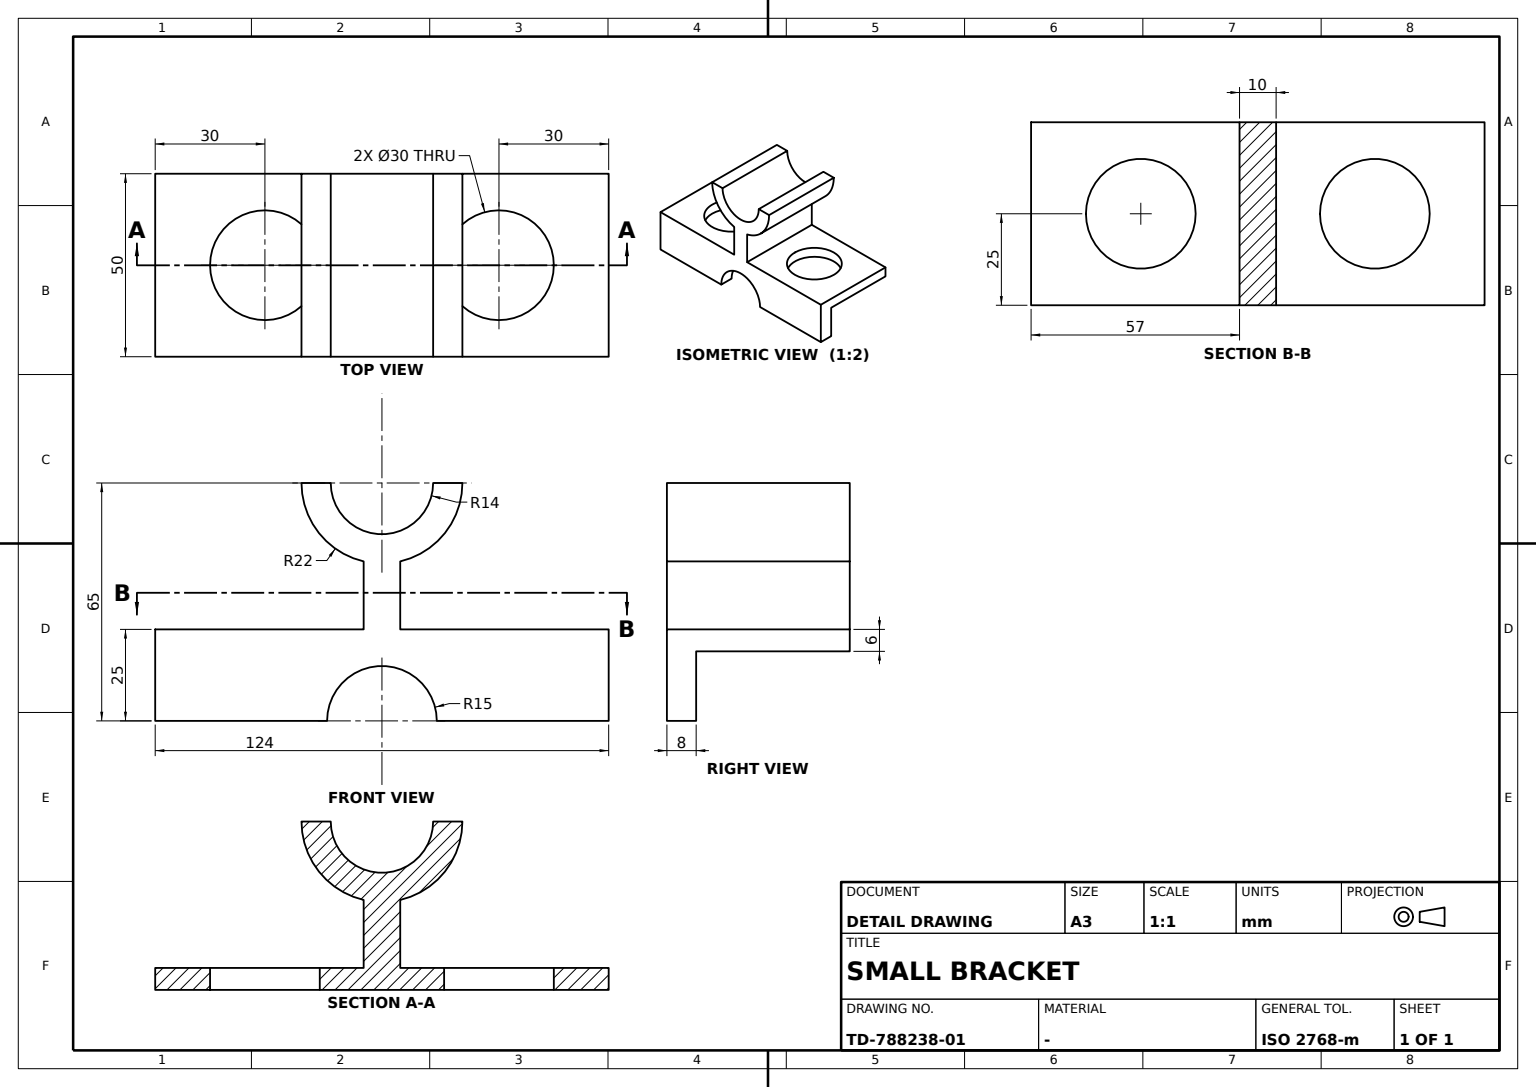
ISO-10303-21;
HEADER;
FILE_DESCRIPTION((''),'2;1');
FILE_NAME('','',(''),(''),'','','');
FILE_SCHEMA(('AUTOMOTIVE_DESIGN'));
ENDSEC;
DATA;
#1=APPLICATION_CONTEXT('');
#2=PRODUCT_CONTEXT('',#1,'mechanical');
#3=PRODUCT('','','',(#2));
#4=PRODUCT_DEFINITION_FORMATION('','',#3);
#5=PRODUCT_DEFINITION_CONTEXT('',#1,'design');
#6=PRODUCT_DEFINITION('','',#4,#5);
#7=PRODUCT_DEFINITION_SHAPE('','',#6);
#8=(LENGTH_UNIT()NAMED_UNIT(*)SI_UNIT(.MILLI.,.METRE.));
#9=(NAMED_UNIT(*)PLANE_ANGLE_UNIT()SI_UNIT($,.RADIAN.));
#10=(NAMED_UNIT(*)SI_UNIT($,.STERADIAN.)SOLID_ANGLE_UNIT());
#11=UNCERTAINTY_MEASURE_WITH_UNIT(LENGTH_MEASURE(0.005),#8,'distance_accuracy_value','');
#12=(GEOMETRIC_REPRESENTATION_CONTEXT(3)GLOBAL_UNCERTAINTY_ASSIGNED_CONTEXT((#11))GLOBAL_UNIT_ASSIGNED_CONTEXT((#8,#9,#10))REPRESENTATION_CONTEXT('',''));
#13=CARTESIAN_POINT('',(-62.,0.,25.));
#14=VERTEX_POINT('',#13);
#15=CARTESIAN_POINT('',(-5.,0.,25.));
#16=VERTEX_POINT('',#15);
#17=CARTESIAN_POINT('',(0.,0.,25.));
#18=DIRECTION('',(1.,0.,0.));
#19=VECTOR('',#18,1000.);
#20=LINE('',#17,#19);
#21=EDGE_CURVE('',#14,#16,#20,.T.);
#22=ORIENTED_EDGE('',*,*,#21,.T.);
#23=CARTESIAN_POINT('',(-5.,50.,25.));
#24=VERTEX_POINT('',#23);
#25=DIRECTION('',(0.,1.,0.));
#26=VECTOR('',#25,1000.);
#27=LINE('',#15,#26);
#28=EDGE_CURVE('',#16,#24,#27,.T.);
#29=ORIENTED_EDGE('',*,*,#28,.T.);
#30=CARTESIAN_POINT('',(-62.,50.,25.));
#31=VERTEX_POINT('',#30);
#32=CARTESIAN_POINT('',(0.,50.,25.));
#33=LINE('',#32,#19);
#34=EDGE_CURVE('',#31,#24,#33,.T.);
#35=ORIENTED_EDGE('',*,*,#34,.F.);
#36=LINE('',#13,#26);
#37=EDGE_CURVE('',#14,#31,#36,.T.);
#38=ORIENTED_EDGE('',*,*,#37,.F.);
#39=EDGE_LOOP('',(#22,#29,#35,#38));
#40=FACE_BOUND('',#39,.T.);
#41=CARTESIAN_POINT('',(-47.,25.,25.));
#42=VERTEX_POINT('',#41);
#43=CARTESIAN_POINT('',(-32.,25.,25.));
#44=DIRECTION('',(0.,0.,-1.));
#45=DIRECTION('',(-1.,0.,0.));
#46=AXIS2_PLACEMENT_3D('',#43,#44,#45);
#47=CIRCLE('',#46,15.);
#48=EDGE_CURVE('',#42,#42,#47,.T.);
#49=ORIENTED_EDGE('',*,*,#48,.T.);
#50=EDGE_LOOP('',(#49));
#51=FACE_BOUND('',#50,.T.);
#52=AXIS2_PLACEMENT_3D('',#17,#44,#25);
#53=PLANE('',#52);
#54=ADVANCED_FACE('',(#40,#51),#53,.F.);
#55=CARTESIAN_POINT('',(5.,50.,25.));
#56=VERTEX_POINT('',#55);
#57=CARTESIAN_POINT('',(62.,50.,25.));
#58=VERTEX_POINT('',#57);
#59=EDGE_CURVE('',#56,#58,#33,.T.);
#60=ORIENTED_EDGE('',*,*,#59,.F.);
#61=CARTESIAN_POINT('',(5.,0.,25.));
#62=VERTEX_POINT('',#61);
#63=LINE('',#61,#26);
#64=EDGE_CURVE('',#62,#56,#63,.T.);
#65=ORIENTED_EDGE('',*,*,#64,.F.);
#66=CARTESIAN_POINT('',(62.,0.,25.));
#67=VERTEX_POINT('',#66);
#68=EDGE_CURVE('',#62,#67,#20,.T.);
#69=ORIENTED_EDGE('',*,*,#68,.T.);
#70=LINE('',#66,#26);
#71=EDGE_CURVE('',#67,#58,#70,.T.);
#72=ORIENTED_EDGE('',*,*,#71,.T.);
#73=EDGE_LOOP('',(#60,#65,#69,#72));
#74=FACE_BOUND('',#73,.T.);
#75=CARTESIAN_POINT('',(17.,25.,25.));
#76=VERTEX_POINT('',#75);
#77=CARTESIAN_POINT('',(32.,25.,25.));
#78=AXIS2_PLACEMENT_3D('',#77,#44,#45);
#79=CIRCLE('',#78,15.);
#80=EDGE_CURVE('',#76,#76,#79,.T.);
#81=ORIENTED_EDGE('',*,*,#80,.T.);
#82=EDGE_LOOP('',(#81));
#83=FACE_BOUND('',#82,.T.);
#84=ADVANCED_FACE('',(#74,#83),#53,.F.);
#85=CARTESIAN_POINT('',(-5.,0.,43.575715));
#86=VERTEX_POINT('',#85);
#87=CARTESIAN_POINT('',(-5.,0.,0.));
#88=DIRECTION('',(0.,0.,1.));
#89=VECTOR('',#88,1000.);
#90=LINE('',#87,#89);
#91=EDGE_CURVE('',#16,#86,#90,.T.);
#92=ORIENTED_EDGE('',*,*,#91,.T.);
#93=CARTESIAN_POINT('',(-5.,50.,43.575715));
#94=VERTEX_POINT('',#93);
#95=DIRECTION('',(0.,-1.,0.));
#96=VECTOR('',#95,1000.);
#97=LINE('',#85,#96);
#98=EDGE_CURVE('',#86,#94,#97,.F.);
#99=ORIENTED_EDGE('',*,*,#98,.T.);
#100=LINE('',#23,#89);
#101=EDGE_CURVE('',#24,#94,#100,.T.);
#102=ORIENTED_EDGE('',*,*,#101,.F.);
#103=ORIENTED_EDGE('',*,*,#28,.F.);
#104=EDGE_LOOP('',(#92,#99,#102,#103));
#105=FACE_BOUND('',#104,.T.);
#106=AXIS2_PLACEMENT_3D('',#15,#45,#88);
#107=PLANE('',#106);
#108=ADVANCED_FACE('',(#105),#107,.T.);
#109=CARTESIAN_POINT('',(-15.,0.,0.));
#110=VERTEX_POINT('',#109);
#111=CARTESIAN_POINT('',(-15.,8.,0.));
#112=VERTEX_POINT('',#111);
#113=LINE('',#111,#96);
#114=EDGE_CURVE('',#110,#112,#113,.F.);
#115=ORIENTED_EDGE('',*,*,#114,.F.);
#116=CARTESIAN_POINT('',(-62.,0.,0.));
#117=VERTEX_POINT('',#116);
#118=CARTESIAN_POINT('',(0.,0.,0.));
#119=LINE('',#118,#19);
#120=EDGE_CURVE('',#117,#110,#119,.T.);
#121=ORIENTED_EDGE('',*,*,#120,.F.);
#122=CARTESIAN_POINT('',(-62.,8.,0.));
#123=VERTEX_POINT('',#122);
#124=LINE('',#116,#96);
#125=EDGE_CURVE('',#123,#117,#124,.T.);
#126=ORIENTED_EDGE('',*,*,#125,.F.);
#127=CARTESIAN_POINT('',(0.,8.,0.));
#128=LINE('',#127,#19);
#129=EDGE_CURVE('',#123,#112,#128,.T.);
#130=ORIENTED_EDGE('',*,*,#129,.T.);
#131=EDGE_LOOP('',(#115,#121,#126,#130));
#132=FACE_BOUND('',#131,.T.);
#133=AXIS2_PLACEMENT_3D('',#127,#88,#95);
#134=PLANE('',#133);
#135=ADVANCED_FACE('',(#132),#134,.F.);
#136=ORIENTED_EDGE('',*,*,#48,.F.);
#137=EDGE_LOOP('',(#136));
#138=FACE_BOUND('',#137,.T.);
#139=CARTESIAN_POINT('',(-17.,25.,19.));
#140=VERTEX_POINT('',#139);
#141=CARTESIAN_POINT('',(-32.,25.,19.));
#142=AXIS2_PLACEMENT_3D('',#141,#88,#18);
#143=CIRCLE('',#142,15.);
#144=EDGE_CURVE('',#140,#140,#143,.T.);
#145=ORIENTED_EDGE('',*,*,#144,.F.);
#146=EDGE_LOOP('',(#145));
#147=FACE_BOUND('',#146,.T.);
#148=CARTESIAN_POINT('',(-32.,25.,24.9));
#149=AXIS2_PLACEMENT_3D('',#148,#44,#18);
#150=CYLINDRICAL_SURFACE('',#149,15.);
#151=ADVANCED_FACE('',(#138,#147),#150,.F.);
#152=CARTESIAN_POINT('',(5.,0.,43.575715));
#153=VERTEX_POINT('',#152);
#154=CARTESIAN_POINT('',(22.,0.,65.));
#155=VERTEX_POINT('',#154);
#156=CARTESIAN_POINT('',(0.,0.,65.));
#157=AXIS2_PLACEMENT_3D('',#156,#25,#88);
#158=CIRCLE('',#157,22.);
#159=EDGE_CURVE('',#153,#155,#158,.F.);
#160=ORIENTED_EDGE('',*,*,#159,.F.);
#161=CARTESIAN_POINT('',(5.,50.,43.575715));
#162=VERTEX_POINT('',#161);
#163=LINE('',#152,#96);
#164=EDGE_CURVE('',#153,#162,#163,.F.);
#165=ORIENTED_EDGE('',*,*,#164,.T.);
#166=CARTESIAN_POINT('',(22.,50.,65.));
#167=VERTEX_POINT('',#166);
#168=CARTESIAN_POINT('',(0.,50.,65.));
#169=AXIS2_PLACEMENT_3D('',#168,#95,#44);
#170=CIRCLE('',#169,22.);
#171=EDGE_CURVE('',#162,#167,#170,.T.);
#172=ORIENTED_EDGE('',*,*,#171,.T.);
#173=LINE('',#154,#96);
#174=EDGE_CURVE('',#155,#167,#173,.F.);
#175=ORIENTED_EDGE('',*,*,#174,.F.);
#176=EDGE_LOOP('',(#160,#165,#172,#175));
#177=FACE_BOUND('',#176,.T.);
#178=CARTESIAN_POINT('',(0.,25.,65.));
#179=AXIS2_PLACEMENT_3D('',#178,#95,#18);
#180=CYLINDRICAL_SURFACE('',#179,22.);
#181=ADVANCED_FACE('',(#177),#180,.T.);
#182=CARTESIAN_POINT('',(15.,0.,0.));
#183=VERTEX_POINT('',#182);
#184=CARTESIAN_POINT('',(62.,0.,0.));
#185=VERTEX_POINT('',#184);
#186=EDGE_CURVE('',#183,#185,#119,.T.);
#187=ORIENTED_EDGE('',*,*,#186,.T.);
#188=LINE('',#184,#89);
#189=EDGE_CURVE('',#185,#67,#188,.T.);
#190=ORIENTED_EDGE('',*,*,#189,.T.);
#191=ORIENTED_EDGE('',*,*,#68,.F.);
#192=CARTESIAN_POINT('',(5.,0.,0.));
#193=LINE('',#192,#89);
#194=EDGE_CURVE('',#62,#153,#193,.T.);
#195=ORIENTED_EDGE('',*,*,#194,.T.);
#196=ORIENTED_EDGE('',*,*,#159,.T.);
#197=CARTESIAN_POINT('',(14.,0.,65.));
#198=VERTEX_POINT('',#197);
#199=LINE('',#156,#19);
#200=EDGE_CURVE('',#198,#155,#199,.T.);
#201=ORIENTED_EDGE('',*,*,#200,.F.);
#202=CARTESIAN_POINT('',(-14.,0.,65.));
#203=VERTEX_POINT('',#202);
#204=CIRCLE('',#157,14.);
#205=EDGE_CURVE('',#203,#198,#204,.F.);
#206=ORIENTED_EDGE('',*,*,#205,.F.);
#207=CARTESIAN_POINT('',(-22.,0.,65.));
#208=VERTEX_POINT('',#207);
#209=EDGE_CURVE('',#208,#203,#199,.T.);
#210=ORIENTED_EDGE('',*,*,#209,.F.);
#211=EDGE_CURVE('',#208,#86,#158,.F.);
#212=ORIENTED_EDGE('',*,*,#211,.T.);
#213=ORIENTED_EDGE('',*,*,#91,.F.);
#214=ORIENTED_EDGE('',*,*,#21,.F.);
#215=LINE('',#116,#89);
#216=EDGE_CURVE('',#117,#14,#215,.T.);
#217=ORIENTED_EDGE('',*,*,#216,.F.);
#218=ORIENTED_EDGE('',*,*,#120,.T.);
#219=AXIS2_PLACEMENT_3D('',#118,#25,#88);
#220=CIRCLE('',#219,15.);
#221=EDGE_CURVE('',#183,#110,#220,.F.);
#222=ORIENTED_EDGE('',*,*,#221,.F.);
#223=EDGE_LOOP('',(#187,#190,#191,#195,#196,#201,#206,#210,#212,#213,#214,#217,#218,#222));
#224=FACE_BOUND('',#223,.T.);
#225=PLANE('',#219);
#226=ADVANCED_FACE('',(#224),#225,.F.);
#227=CARTESIAN_POINT('',(47.,25.,19.));
#228=VERTEX_POINT('',#227);
#229=CARTESIAN_POINT('',(32.,25.,19.));
#230=AXIS2_PLACEMENT_3D('',#229,#88,#18);
#231=CIRCLE('',#230,15.);
#232=EDGE_CURVE('',#228,#228,#231,.T.);
#233=ORIENTED_EDGE('',*,*,#232,.T.);
#234=EDGE_LOOP('',(#233));
#235=FACE_BOUND('',#234,.T.);
#236=CARTESIAN_POINT('',(-62.,50.,19.));
#237=VERTEX_POINT('',#236);
#238=CARTESIAN_POINT('',(-62.,8.,19.));
#239=VERTEX_POINT('',#238);
#240=CARTESIAN_POINT('',(-62.,0.,19.));
#241=LINE('',#240,#96);
#242=EDGE_CURVE('',#237,#239,#241,.T.);
#243=ORIENTED_EDGE('',*,*,#242,.F.);
#244=CARTESIAN_POINT('',(62.,50.,19.));
#245=VERTEX_POINT('',#244);
#246=CARTESIAN_POINT('',(0.,50.,19.));
#247=LINE('',#246,#19);
#248=EDGE_CURVE('',#237,#245,#247,.T.);
#249=ORIENTED_EDGE('',*,*,#248,.T.);
#250=CARTESIAN_POINT('',(62.,8.,19.));
#251=VERTEX_POINT('',#250);
#252=CARTESIAN_POINT('',(62.,0.,19.));
#253=LINE('',#252,#96);
#254=EDGE_CURVE('',#245,#251,#253,.T.);
#255=ORIENTED_EDGE('',*,*,#254,.T.);
#256=CARTESIAN_POINT('',(0.,8.,19.));
#257=LINE('',#256,#19);
#258=EDGE_CURVE('',#239,#251,#257,.T.);
#259=ORIENTED_EDGE('',*,*,#258,.F.);
#260=EDGE_LOOP('',(#243,#249,#255,#259));
#261=FACE_BOUND('',#260,.T.);
#262=ORIENTED_EDGE('',*,*,#144,.T.);
#263=EDGE_LOOP('',(#262));
#264=FACE_BOUND('',#263,.T.);
#265=AXIS2_PLACEMENT_3D('',#246,#88,#95);
#266=PLANE('',#265);
#267=ADVANCED_FACE('',(#235,#261,#264),#266,.F.);
#268=ORIENTED_EDGE('',*,*,#129,.F.);
#269=VECTOR('',#44,1000.);
#270=LINE('',#122,#269);
#271=EDGE_CURVE('',#239,#123,#270,.T.);
#272=ORIENTED_EDGE('',*,*,#271,.F.);
#273=ORIENTED_EDGE('',*,*,#258,.T.);
#274=CARTESIAN_POINT('',(62.,8.,0.));
#275=VERTEX_POINT('',#274);
#276=LINE('',#274,#269);
#277=EDGE_CURVE('',#251,#275,#276,.T.);
#278=ORIENTED_EDGE('',*,*,#277,.T.);
#279=CARTESIAN_POINT('',(15.,8.,0.));
#280=VERTEX_POINT('',#279);
#281=EDGE_CURVE('',#280,#275,#128,.T.);
#282=ORIENTED_EDGE('',*,*,#281,.F.);
#283=AXIS2_PLACEMENT_3D('',#127,#95,#44);
#284=CIRCLE('',#283,15.);
#285=EDGE_CURVE('',#280,#112,#284,.T.);
#286=ORIENTED_EDGE('',*,*,#285,.T.);
#287=EDGE_LOOP('',(#268,#272,#273,#278,#282,#286));
#288=FACE_BOUND('',#287,.T.);
#289=AXIS2_PLACEMENT_3D('',#256,#95,#44);
#290=PLANE('',#289);
#291=ADVANCED_FACE('',(#288),#290,.F.);
#292=ORIENTED_EDGE('',*,*,#114,.T.);
#293=ORIENTED_EDGE('',*,*,#285,.F.);
#294=LINE('',#279,#96);
#295=EDGE_CURVE('',#280,#183,#294,.T.);
#296=ORIENTED_EDGE('',*,*,#295,.T.);
#297=ORIENTED_EDGE('',*,*,#221,.T.);
#298=EDGE_LOOP('',(#292,#293,#296,#297));
#299=FACE_BOUND('',#298,.T.);
#300=CARTESIAN_POINT('',(0.,25.66,0.));
#301=AXIS2_PLACEMENT_3D('',#300,#95,#18);
#302=CYLINDRICAL_SURFACE('',#301,15.);
#303=ADVANCED_FACE('',(#299),#302,.F.);
#304=CARTESIAN_POINT('',(-22.,50.,65.));
#305=VERTEX_POINT('',#304);
#306=CARTESIAN_POINT('',(-14.,50.,65.));
#307=VERTEX_POINT('',#306);
#308=LINE('',#304,#19);
#309=EDGE_CURVE('',#305,#307,#308,.T.);
#310=ORIENTED_EDGE('',*,*,#309,.F.);
#311=LINE('',#207,#96);
#312=EDGE_CURVE('',#208,#305,#311,.F.);
#313=ORIENTED_EDGE('',*,*,#312,.F.);
#314=ORIENTED_EDGE('',*,*,#209,.T.);
#315=LINE('',#202,#96);
#316=EDGE_CURVE('',#203,#307,#315,.F.);
#317=ORIENTED_EDGE('',*,*,#316,.T.);
#318=EDGE_LOOP('',(#310,#313,#314,#317));
#319=FACE_BOUND('',#318,.T.);
#320=AXIS2_PLACEMENT_3D('',#207,#88,#18);
#321=PLANE('',#320);
#322=ADVANCED_FACE('',(#319),#321,.T.);
#323=ORIENTED_EDGE('',*,*,#186,.F.);
#324=ORIENTED_EDGE('',*,*,#295,.F.);
#325=ORIENTED_EDGE('',*,*,#281,.T.);
#326=LINE('',#184,#96);
#327=EDGE_CURVE('',#275,#185,#326,.T.);
#328=ORIENTED_EDGE('',*,*,#327,.T.);
#329=EDGE_LOOP('',(#323,#324,#325,#328));
#330=FACE_BOUND('',#329,.T.);
#331=ADVANCED_FACE('',(#330),#134,.F.);
#332=CARTESIAN_POINT('',(14.,50.,65.));
#333=VERTEX_POINT('',#332);
#334=EDGE_CURVE('',#333,#167,#308,.T.);
#335=ORIENTED_EDGE('',*,*,#334,.F.);
#336=LINE('',#197,#96);
#337=EDGE_CURVE('',#198,#333,#336,.F.);
#338=ORIENTED_EDGE('',*,*,#337,.F.);
#339=ORIENTED_EDGE('',*,*,#200,.T.);
#340=ORIENTED_EDGE('',*,*,#174,.T.);
#341=EDGE_LOOP('',(#335,#338,#339,#340));
#342=FACE_BOUND('',#341,.T.);
#343=ADVANCED_FACE('',(#342),#321,.T.);
#344=ORIENTED_EDGE('',*,*,#64,.T.);
#345=LINE('',#55,#89);
#346=EDGE_CURVE('',#56,#162,#345,.T.);
#347=ORIENTED_EDGE('',*,*,#346,.T.);
#348=ORIENTED_EDGE('',*,*,#164,.F.);
#349=ORIENTED_EDGE('',*,*,#194,.F.);
#350=EDGE_LOOP('',(#344,#347,#348,#349));
#351=FACE_BOUND('',#350,.T.);
#352=AXIS2_PLACEMENT_3D('',#61,#45,#88);
#353=PLANE('',#352);
#354=ADVANCED_FACE('',(#351),#353,.F.);
#355=ORIENTED_EDGE('',*,*,#316,.F.);
#356=ORIENTED_EDGE('',*,*,#205,.T.);
#357=ORIENTED_EDGE('',*,*,#337,.T.);
#358=CIRCLE('',#169,14.);
#359=EDGE_CURVE('',#307,#333,#358,.T.);
#360=ORIENTED_EDGE('',*,*,#359,.F.);
#361=EDGE_LOOP('',(#355,#356,#357,#360));
#362=FACE_BOUND('',#361,.T.);
#363=CYLINDRICAL_SURFACE('',#179,14.);
#364=ADVANCED_FACE('',(#362),#363,.F.);
#365=EDGE_CURVE('',#305,#94,#170,.T.);
#366=ORIENTED_EDGE('',*,*,#365,.T.);
#367=ORIENTED_EDGE('',*,*,#98,.F.);
#368=ORIENTED_EDGE('',*,*,#211,.F.);
#369=ORIENTED_EDGE('',*,*,#312,.T.);
#370=EDGE_LOOP('',(#366,#367,#368,#369));
#371=FACE_BOUND('',#370,.T.);
#372=ADVANCED_FACE('',(#371),#180,.T.);
#373=ORIENTED_EDGE('',*,*,#365,.F.);
#374=ORIENTED_EDGE('',*,*,#309,.T.);
#375=ORIENTED_EDGE('',*,*,#359,.T.);
#376=ORIENTED_EDGE('',*,*,#334,.T.);
#377=ORIENTED_EDGE('',*,*,#171,.F.);
#378=ORIENTED_EDGE('',*,*,#346,.F.);
#379=ORIENTED_EDGE('',*,*,#59,.T.);
#380=CARTESIAN_POINT('',(62.,50.,0.));
#381=LINE('',#380,#269);
#382=EDGE_CURVE('',#58,#245,#381,.T.);
#383=ORIENTED_EDGE('',*,*,#382,.T.);
#384=ORIENTED_EDGE('',*,*,#248,.F.);
#385=CARTESIAN_POINT('',(-62.,50.,0.));
#386=LINE('',#385,#269);
#387=EDGE_CURVE('',#31,#237,#386,.T.);
#388=ORIENTED_EDGE('',*,*,#387,.F.);
#389=ORIENTED_EDGE('',*,*,#34,.T.);
#390=ORIENTED_EDGE('',*,*,#101,.T.);
#391=EDGE_LOOP('',(#373,#374,#375,#376,#377,#378,#379,#383,#384,#388,#389,#390));
#392=FACE_BOUND('',#391,.T.);
#393=AXIS2_PLACEMENT_3D('',#32,#95,#44);
#394=PLANE('',#393);
#395=ADVANCED_FACE('',(#392),#394,.F.);
#396=ORIENTED_EDGE('',*,*,#382,.F.);
#397=ORIENTED_EDGE('',*,*,#71,.F.);
#398=ORIENTED_EDGE('',*,*,#189,.F.);
#399=ORIENTED_EDGE('',*,*,#327,.F.);
#400=ORIENTED_EDGE('',*,*,#277,.F.);
#401=ORIENTED_EDGE('',*,*,#254,.F.);
#402=EDGE_LOOP('',(#396,#397,#398,#399,#400,#401));
#403=FACE_BOUND('',#402,.T.);
#404=AXIS2_PLACEMENT_3D('',#184,#18,#25);
#405=PLANE('',#404);
#406=ADVANCED_FACE('',(#403),#405,.T.);
#407=ORIENTED_EDGE('',*,*,#387,.T.);
#408=ORIENTED_EDGE('',*,*,#242,.T.);
#409=ORIENTED_EDGE('',*,*,#271,.T.);
#410=ORIENTED_EDGE('',*,*,#125,.T.);
#411=ORIENTED_EDGE('',*,*,#216,.T.);
#412=ORIENTED_EDGE('',*,*,#37,.T.);
#413=EDGE_LOOP('',(#407,#408,#409,#410,#411,#412));
#414=FACE_BOUND('',#413,.T.);
#415=AXIS2_PLACEMENT_3D('',#116,#18,#25);
#416=PLANE('',#415);
#417=ADVANCED_FACE('',(#414),#416,.F.);
#418=ORIENTED_EDGE('',*,*,#80,.F.);
#419=EDGE_LOOP('',(#418));
#420=FACE_BOUND('',#419,.T.);
#421=ORIENTED_EDGE('',*,*,#232,.F.);
#422=EDGE_LOOP('',(#421));
#423=FACE_BOUND('',#422,.T.);
#424=CARTESIAN_POINT('',(32.,25.,24.9));
#425=AXIS2_PLACEMENT_3D('',#424,#44,#18);
#426=CYLINDRICAL_SURFACE('',#425,15.);
#427=ADVANCED_FACE('',(#420,#423),#426,.F.);
#428=CLOSED_SHELL('',(#54,#84,#108,#135,#151,#181,#226,#267,#291,#303,#322,#331,#343,#354,#364,#372,#395,#406,#417,#427));
#429=MANIFOLD_SOLID_BREP('',#428);
#430=ADVANCED_BREP_SHAPE_REPRESENTATION('',(#429),#12);
#431=SHAPE_DEFINITION_REPRESENTATION(#7,#430);
ENDSEC;
END-ISO-10303-21;
